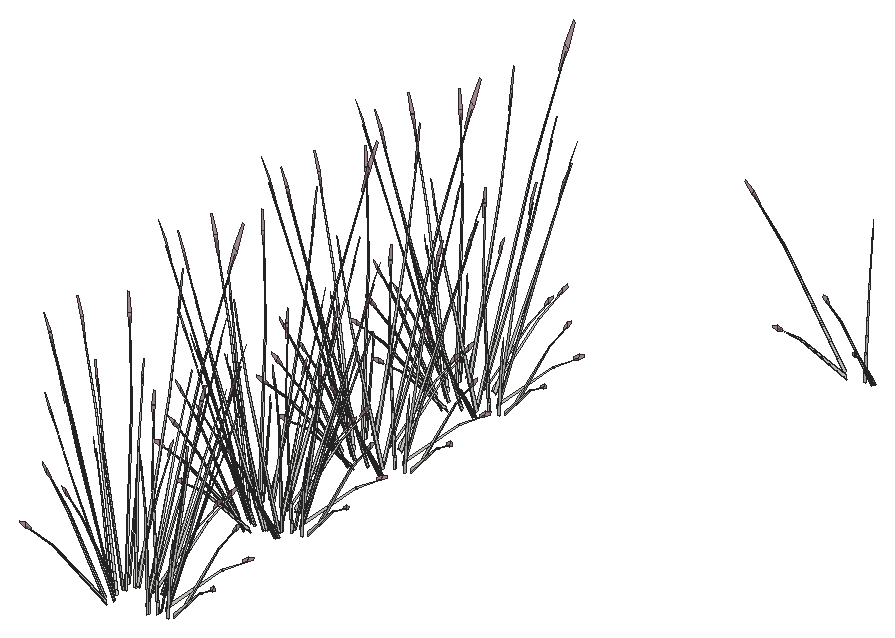
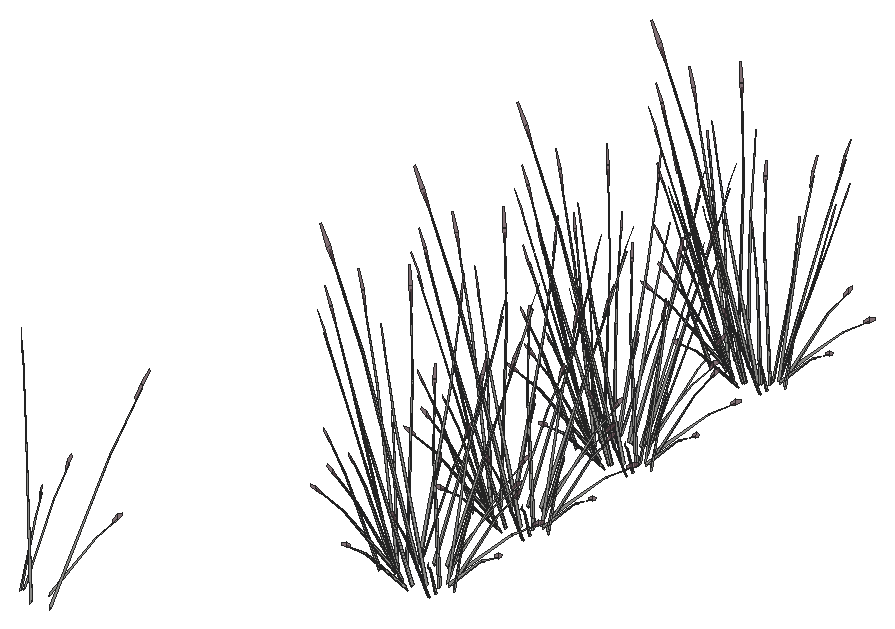
# SketchUp Ruby script. Lengths in inches.
U = 1.inch
M = Sketchup.active_model
def pt(a) = Geom::Point3d.new(a.map { |v| v * U })
def face(e, loops, mat)
  f = e.add_face(loops[0].map { |a| pt(a) })
  loops[1..].each { |l| e.add_face(l.map { |a| pt(a) }).erase! }
  f.material = f.back_material = mat if mat
  f
end
# faces: each face lists its corners as indices into pts; further lists are holes
def faces(e, pts, list, mat = nil) = list.each { |f| face(e, (f[0].is_a?(Array) ? f : [f]).map { |l| l.map { |i| pts[i] } }, mat) }
# xy, xz, yz: faces in a plane at the given z, y or x. An outline is a flat list of corners, or four numbers for a rectangle; further outlines are holes
def ring(l) = l.size == 4 ? [[l[0], l[1]], [l[2], l[1]], [l[2], l[3]], [l[0], l[3]]] : l.each_slice(2).to_a
def flat(e, list, mat, &to3) = list.each { |f| face(e, (f[0].is_a?(Array) ? f : [f]).map { |l| ring(l).map { |u, v| to3.(u, v) } }, mat) }
def xy(e, z, list, mat = nil) = flat(e, list, mat) { |x, y| [x, y, z] }
def xz(e, y, list, mat = nil) = flat(e, list, mat) { |x, z| [x, y, z] }
def yz(e, x, list, mat = nil) = flat(e, list, mat) { |y, z| [x, y, z] }
def lines(e, pts, list) = list.each { |a, b| e.add_line(pt(pts[a]), pt(pts[b])) }
# prism: a flat outline (further loops are holes) pulled along v
def prism(e, loops, v, mat = nil)
  f = face(e, loops, mat); d = Geom::Vector3d.new(v.map { |x| x * U })
  f.pushpull(f.normal.samedirection?(d) ? d.length : -d.length)
end
def box(e, o, s, mat = nil) = prism(e, [[o, [o[0] + s[0], o[1], o[2]], [o[0] + s[0], o[1] + s[1], o[2]], [o[0], o[1] + s[1], o[2]]]], [0, 0, s[2]], mat)
def at(x, y, z, deg = 0) = Geom::Transformation.translation(pt([x, y, z])) * Geom::Transformation.rotation(ORIGIN, Z_AXIS, deg.degrees)
def axes(o, x, y, z) = Geom::Transformation.new([*x, 0, *y, 0, *z, 0, *pt(o).to_a, 1])
def part(name) = M.definitions.add(name)
# library, detail: a bought-in or finely detailed component or shape, given as its bounding box
def library(name, o, s) = part(name).tap { |d| box(d.entities, o, s) }
def detail(e, o, s) = box(e.add_group.entities, o, s)
def put(e, d, t, mat = nil) = e.add_instance(d, t).tap { |i| i.material = mat if mat }
def group(e, t, mat = nil) = e.add_group.tap { |g| g.transformation = t; g.material = mat if mat }.entities
root = M.entities
M.materials.add("LightPink_Translucent").color = [144, 107, 117]
M.materials["LightPink_Translucent"].alpha = 0.75
c1 = part("blade")
p = [[2.15,0.21,22],[0,0.17,0],[0.09,0.45,0],[2.18,0.31,22],[2.29,0.31,22],[0.38,0.45,0],
  [2.48,0.24,33],[2.49,0.24,33],[2.48,0.22,33]]
faces(c1.entities,p,[[0,1,2,3],[4,5,2,3],[6,3,4,7],[8,0,3,6]])
c2 = part("seeds")
p = [[0.3,-0.1,1.38],[-0.01,-0.03,1.59],[-0.01,-0.03,0.03],[0.14,-0.07,-0.07],[0.29,-0.03,3],[0.15,0.01,3.11]]
faces(c2.entities,p,[[0,1,2,3],[1,0,4,5]],"LightPink_Translucent")
c3 = part("blade with seeds")
put(c3.entities,c1,at(0,0,0))
put(c3.entities,c2,axes([2.4,0.25,30.99],[1.5799,-0.05474,1.17369],[-0.12525,1.92788,0.29478],[-0.07173,-0.02425,1.56792]))
put(root,c3,axes([673.85,236.19,513.93],[0.53464,0.0266,0.05337],[-0.01466,0.40172,0.42015],[0.05594,-0.15388,0.64067]))
put(root,c3,axes([669.22,235.43,513.91],[-0.13998,-0.00403,1.45204],[-0.44565,0.40302,-0.22964],[-0.23779,-0.08235,0.11645]))
put(root,c3,axes([674.51,237.4375,514.18],[-0.60181,-0.31483,-0.10093],[0.34671,-0.45593,-0.56021],[0.17003,-0.15849,0.85122]))
put(root,c3,axes([675.99,237.3,513.91],[-0.08498,-0.00434,1.47228],[-0.35287,-0.46464,-0.13912],[0.14171,-0.15278,0.26054]))
put(root,c3,axes([669.37,236.34,513.93],[0.03276,-0.43418,0.05337],[0.49468,0.0119,0.42015],[-0.18949,-0.04543,0.64067]))
put(root,c3,axes([674.73,237.32,513.93],[0.44663,0.24013,0.05337],[-0.26003,0.34195,0.42015],[0.14319,-0.11055,0.64067]))
put(root,c3,axes([676.32,237.86,513.91],[0.09028,-0.08697,1.45204],[-0.11555,-0.53348,-0.22964],[0.22652,-0.10115,0.11645]))
put(root,c3,axes([668.6875,235.77,513.91],[0.04823,0.05698,1.47228],[-0.23252,0.51221,-0.13912],[-0.23548,0.00371,0.26054]))
put(root,c3,axes([669.6,236.4375,514.18],[-0.03484,0.58066,-0.10093],[-0.65957,-0.01587,-0.56021],[-0.25402,-0.04034,0.85122]))
put(root,c3,axes([674.54,238.67,514.18],[-0.32734,-0.51701,-0.10093],[0.58097,-0.25407,-0.56021],[0.24483,-0.06821,0.85122]))
put(root,c3,axes([668.6,237.52,513.93],[-0.23895,-0.38931,0.05337],[0.43573,-0.19055,0.42015],[-0.19208,0.0376,0.64067]))
put(root,c3,axes([674.8,238.65,513.93],[0.23895,0.38931,0.05337],[-0.43573,0.19055,0.42015],[0.19208,-0.0376,0.64067]))
put(root,c3,axes([675.84,240.2,513.91],[-0.05883,-0.04999,1.47228],[0.12868,-0.53581,-0.13912],[0.23172,-0.03423,0.26054]))
put(root,c3,axes([668.18,238.03,513.91],[-0.10624,0.07413,1.45204],[0.00904,0.54162,-0.22964],[-0.24352,0.07044,0.11645]))
put(root,c3,axes([668.87,237.51,514.18],[0.32734,0.51701,-0.10093],[-0.58097,0.25407,-0.56021],[-0.24483,0.06821,0.85122]))
put(root,c3,axes([673.8,239.74,514.18],[0.03484,-0.58066,-0.10093],[0.65957,0.01587,-0.56021],[0.25402,0.04034,0.85122]))
put(root,c3,axes([674.375,239.39,513.91],[0.13956,-0.00966,1.45204],[0.38281,-0.44358,-0.22964],[0.24825,0.05855,0.11645]))
put(root,c3,axes([668.67,238.86,513.93],[-0.44663,-0.24013,0.05337],[0.26003,-0.34195,0.42015],[-0.14319,0.11055,0.64067]))
put(root,c3,axes([667,238.57,513.91],[0.08303,0.01531,1.47228],[0.25685,0.50448,-0.13912],[-0.16996,0.13241,0.26054]))
put(root,c3,axes([674.04,239.84,513.93],[-0.03276,0.43418,0.05337],[-0.49468,-0.0119,0.42015],[0.18949,0.04543,0.64067]))
put(root,c3,axes([672.94,237.49,513.71],[-0.56218,-0.29666,1.14775],[0.59361,-0.46189,0.49522],[0.18138,0.27836,1.10941]))
put(root,c3,axes([668.89,238.74,514.18],[0.60181,0.31483,-0.10093],[-0.34671,0.45593,-0.56021],[-0.17003,0.15849,0.85122]))
put(root,c3,axes([672.5,240.37,514.18],[0.38768,-0.48872,-0.10093],[0.56143,0.28156,-0.56021],[0.19516,0.13808,0.85122]))
put(root,c3,axes([672,240.78,513.91],[0.00193,-0.06913,1.47228],[0.55753,-0.30498,-0.13912],[0.19366,0.10886,0.26054]))
put(root,c3,axes([669.55,239.98,513.93],[-0.53464,-0.0266,0.05337],[0.01466,-0.40172,0.42015],[-0.05594,0.15388,0.64067]))
put(root,c3,axes([672.65,240.55,513.93],[-0.29569,0.36271,0.05337],[-0.42107,-0.21117,0.42015],[0.13613,0.11629,0.64067]))
put(root,c3,axes([671,240.6,513.93],[-0.47939,0.19405,0.05337],[-0.23464,-0.35385,0.42015],[0.0463,0.15598,0.64067]))
put(root,c3,axes([668.2,240.05,513.91],[-0.01617,0.11299,1.45204],[0.45894,0.39307,-0.22964],[-0.12015,0.18588,0.11645]))
put(root,c3,axes([669.67,239.79,514.48],[0.71502,0.02829,-0.11203],[-0.01954,0.53563,-0.62183],[-0.04967,0.20629,0.94486]))
put(root,c3,axes([670.99,240.39,514.18],[0.63664,-0.26583,-0.10093],[0.31286,0.47181,-0.56021],[0.084,0.19882,0.85122]))
put(root,c3,axes([668.15,241.21,513.91],[0.07381,-0.03447,1.47228],[0.61004,0.22929,-0.13912],[-0.01434,0.19091,0.26054]))
put(root,c3,axes([670.84,241.45,513.91],[0.08247,0.09194,1.45204],[0.66552,0.03612,-0.22964],[0.06692,0.20277,0.11645]))
put(root,c3,axes([671.4,256.4,513.91],[-0.09951,-0.08005,1.45204],[-0.66407,0.05075,-0.22964],[-0.10598,-0.19148,0.11645]))
put(root,c3,axes([674.39,257.375,513.91],[-0.00628,-0.11364,1.45204],[-0.53042,-0.32843,-0.22964],[0.08201,-0.19909,0.11645]))
put(root,c3,axes([674.24,256.97,513.91],[-0.06607,0.04361,1.47228],[-0.64734,-0.14714,-0.13912],[-0.02343,-0.19032,0.26054]))
put(root,c3,axes([670.72,256.13,513.91],[-0.01214,0.06844,1.47228],[-0.59861,0.24837,-0.13912],[-0.17615,-0.12696,0.26054]))
put(root,c3,axes([672.41,257.63,514.18],[-0.63664,0.26583,-0.10093],[-0.31286,-0.47181,-0.56021],[-0.084,-0.19882,0.85122]))
put(root,c3,axes([673.74,258.23,514.18],[-0.71502,-0.02829,-0.10093],[0.01954,-0.53563,-0.56021],[0.04967,-0.20629,0.85122]))
put(root,c3,axes([672.4,257.42,513.93],[0.47939,-0.19405,0.05337],[0.23464,0.35385,0.42015],[-0.0463,-0.15598,0.64067]))
put(root,c3,axes([670.76,257.47,513.93],[0.29569,-0.36271,0.05337],[0.42107,0.21117,0.42015],[-0.13613,-0.11629,0.64067]))
put(root,c3,axes([670.89,257.43,514.51],[-0.4342,0.54737,-0.11304],[-0.6288,-0.31535,-0.62743],[-0.21858,-0.15465,0.95337]))
put(root,c3,axes([673.85,258.04,513.93],[0.53464,0.0266,0.05337],[-0.01466,0.40172,0.42015],[0.05594,-0.15388,0.64067]))
put(root,c3,axes([669.22,257.28,513.91],[-0.13998,-0.00403,1.45204],[-0.44565,0.40302,-0.22964],[-0.23779,-0.08235,0.11645]))
put(root,c3,axes([674.51,259.28,514.18],[-0.60181,-0.31483,-0.10093],[0.34671,-0.45593,-0.56021],[0.17003,-0.15849,0.85122]))
put(root,c3,axes([675.99,259.15,513.91],[-0.08498,-0.00434,1.47228],[-0.35287,-0.46464,-0.13912],[0.14171,-0.15278,0.26054]))
put(root,c3,axes([669.37,258.19,513.93],[0.03276,-0.43418,0.05337],[0.49468,0.0119,0.42015],[-0.18949,-0.04543,0.64067]))
put(root,c3,axes([674.73,259.17,513.93],[0.44663,0.24013,0.05337],[-0.26003,0.34195,0.42015],[0.14319,-0.11055,0.64067]))
put(root,c3,axes([676.32,259.7,513.91],[0.09028,-0.08697,1.45204],[-0.11555,-0.53348,-0.22964],[0.22652,-0.10115,0.11645]))
put(root,c3,axes([668.6875,257.62,513.91],[0.04823,0.05698,1.47228],[-0.23252,0.51221,-0.13912],[-0.23548,0.00371,0.26054]))
put(root,c3,axes([669.6,258.28,514.18],[-0.03484,0.58066,-0.10093],[-0.65957,-0.01587,-0.56021],[-0.25402,-0.04034,0.85122]))
put(root,c3,axes([674.54,260.51,514.18],[-0.32734,-0.51701,-0.10093],[0.58097,-0.25407,-0.56021],[0.24483,-0.06821,0.85122]))
put(root,c3,axes([674.8,260.5,513.93],[0.23895,0.38931,0.05337],[-0.43573,0.19055,0.42015],[0.19208,-0.0376,0.64067]))
put(root,c3,axes([675.84,262.05,513.91],[-0.05883,-0.04999,1.47228],[0.12868,-0.53581,-0.13912],[0.23172,-0.03423,0.26054]))
put(root,c3,axes([668.18,259.87,513.91],[-0.10624,0.07413,1.45204],[0.00904,0.54162,-0.22964],[-0.24352,0.07044,0.11645]))
put(root,c3,axes([668.87,259.36,514.18],[0.32734,0.51701,-0.10093],[-0.58097,0.25407,-0.56021],[-0.24483,0.06821,0.85122]))
put(root,c3,axes([673.8,261.58,514.18],[0.03484,-0.58066,-0.10093],[0.65957,0.01587,-0.56021],[0.25402,0.04034,0.85122]))
put(root,c3,axes([674.375,261.24,513.91],[0.13956,-0.00966,1.45204],[0.38281,-0.44358,-0.22964],[0.24825,0.05855,0.11645]))
put(root,c3,axes([668.67,260.7,513.93],[-0.44663,-0.24013,0.05337],[0.26003,-0.34195,0.42015],[-0.14319,0.11055,0.64067]))
put(root,c3,axes([667,260.42,513.91],[0.08303,0.01531,1.47228],[0.25685,0.50448,-0.13912],[-0.16996,0.13241,0.26054]))
put(root,c3,axes([674.04,261.68,513.93],[-0.03276,0.43418,0.05337],[-0.49468,-0.0119,0.42015],[0.18949,0.04543,0.64067]))
put(root,c3,axes([672.94,259.33,513.71],[-0.56218,-0.29666,1.14775],[0.59361,-0.46189,0.49522],[0.18138,0.27836,1.10941]))
put(root,c3,axes([668.89,260.58,514.18],[0.60181,0.31483,-0.10093],[-0.34671,0.45593,-0.56021],[-0.17003,0.15849,0.85122]))
put(root,c3,axes([672.5,262.22,514.18],[0.38768,-0.48872,-0.10093],[0.56143,0.28156,-0.56021],[0.19516,0.13808,0.85122]))
put(root,c3,axes([672,262.62,513.91],[0.00193,-0.06913,1.47228],[0.55753,-0.30498,-0.13912],[0.19366,0.10886,0.26054]))
put(root,c3,axes([671,262.45,513.93],[-0.47939,0.19405,0.05337],[-0.23464,-0.35385,0.42015],[0.0463,0.15598,0.64067]))
put(root,c3,axes([668.2,261.89,513.91],[-0.01617,0.11299,1.45204],[0.45894,0.39307,-0.22964],[-0.12015,0.18588,0.11645]))
put(root,c3,axes([669.67,261.64,514.48],[0.71502,0.02829,-0.11203],[-0.01954,0.53563,-0.62183],[-0.04967,0.20629,0.94486]))
put(root,c3,axes([670.99,262.24,514.18],[0.63664,-0.26583,-0.10093],[0.31286,0.47181,-0.56021],[0.084,0.19882,0.85122]))
put(root,c3,axes([668.15,263.05,513.91],[0.07381,-0.03447,1.47228],[0.61004,0.22929,-0.13912],[-0.01434,0.19091,0.26054]))
put(root,c3,axes([670.84,263.29,513.91],[0.08247,0.09194,1.45204],[0.66552,0.03612,-0.22964],[0.06692,0.20277,0.11645]))
put(root,c3,axes([671.4,273.25,513.91],[-0.09951,-0.08005,1.45204],[-0.66407,0.05075,-0.22964],[-0.10598,-0.19148,0.11645]))
put(root,c3,axes([674.39,274.24,513.91],[-0.00628,-0.11364,1.45204],[-0.53042,-0.32843,-0.22964],[0.08201,-0.19909,0.11645]))
put(root,c3,axes([674.24,273.83,513.91],[-0.06607,0.04361,1.47228],[-0.64734,-0.14714,-0.13912],[-0.02343,-0.19032,0.26054]))
put(root,c3,axes([670.72,272.99,513.91],[-0.01214,0.06844,1.47228],[-0.59861,0.24837,-0.13912],[-0.17615,-0.12696,0.26054]))
put(root,c3,axes([672.41,274.49,514.18],[-0.63664,0.26583,-0.10093],[-0.31286,-0.47181,-0.56021],[-0.084,-0.19882,0.85122]))
put(root,c3,axes([673.74,275.09,514.18],[-0.71502,-0.02829,-0.10093],[0.01954,-0.53563,-0.56021],[0.04967,-0.20629,0.85122]))
put(root,c3,axes([670.89,274.29,514.51],[-0.4342,0.54737,-0.11304],[-0.6288,-0.31535,-0.62743],[-0.21858,-0.15465,0.95337]))
put(root,c3,axes([669.22,274.14,513.91],[-0.13998,-0.00403,1.45204],[-0.44565,0.40302,-0.22964],[-0.23779,-0.08235,0.11645]))
put(root,c3,axes([674.51,276.14,514.18],[-0.60181,-0.31483,-0.10093],[0.34671,-0.45593,-0.56021],[0.17003,-0.15849,0.85122]))
put(root,c3,axes([675.99,276,513.91],[-0.08498,-0.00434,1.47228],[-0.35287,-0.46464,-0.13912],[0.14171,-0.15278,0.26054]))
put(root,c3,axes([676.32,276.56,513.91],[0.09028,-0.08697,1.45204],[-0.11555,-0.53348,-0.22964],[0.22652,-0.10115,0.11645]))
put(root,c3,axes([668.6875,274.48,513.91],[0.04823,0.05698,1.47228],[-0.23252,0.51221,-0.13912],[-0.23548,0.00371,0.26054]))
put(root,c3,axes([669.6,275.14,514.18],[-0.03484,0.58066,-0.10093],[-0.65957,-0.01587,-0.56021],[-0.25402,-0.04034,0.85122]))
put(root,c3,axes([674.54,277.37,514.18],[-0.32734,-0.51701,-0.10093],[0.58097,-0.25407,-0.56021],[0.24483,-0.06821,0.85122]))
put(root,c3,axes([675.84,278.91,513.91],[-0.05883,-0.04999,1.47228],[0.12868,-0.53581,-0.13912],[0.23172,-0.03423,0.26054]))
put(root,c3,axes([668.18,276.73,513.91],[-0.10624,0.07413,1.45204],[0.00904,0.54162,-0.22964],[-0.24352,0.07044,0.11645]))
put(root,c3,axes([668.87,276.22,514.18],[0.32734,0.51701,-0.10093],[-0.58097,0.25407,-0.56021],[-0.24483,0.06821,0.85122]))
put(root,c3,axes([673.8,278.44,514.18],[0.03484,-0.58066,-0.10093],[0.65957,0.01587,-0.56021],[0.25402,0.04034,0.85122]))
put(root,c3,axes([674.375,278.1,513.91],[0.13956,-0.00966,1.45204],[0.38281,-0.44358,-0.22964],[0.24825,0.05855,0.11645]))
put(root,c3,axes([667,277.28,513.91],[0.08303,0.01531,1.47228],[0.25685,0.50448,-0.13912],[-0.16996,0.13241,0.26054]))
put(root,c3,axes([672.94,276.19,513.71],[-0.56218,-0.29666,1.14775],[0.59361,-0.46189,0.49522],[0.18138,0.27836,1.10941]))
put(root,c3,axes([668.89,277.44,514.18],[0.60181,0.31483,-0.10093],[-0.34671,0.45593,-0.56021],[-0.17003,0.15849,0.85122]))
put(root,c3,axes([672.5,279.08,514.18],[0.38768,-0.48872,-0.10093],[0.56143,0.28156,-0.56021],[0.19516,0.13808,0.85122]))
put(root,c3,axes([672,279.48,513.91],[0.00193,-0.06913,1.47228],[0.55753,-0.30498,-0.13912],[0.19366,0.10886,0.26054]))
put(root,c3,axes([668.2,278.75,513.91],[-0.01617,0.11299,1.45204],[0.45894,0.39307,-0.22964],[-0.12015,0.18588,0.11645]))
put(root,c3,axes([669.67,278.5,514.48],[0.71502,0.02829,-0.11203],[-0.01954,0.53563,-0.62183],[-0.04967,0.20629,0.94486]))
put(root,c3,axes([670.99,279.1,514.18],[0.63664,-0.26583,-0.10093],[0.31286,0.47181,-0.56021],[0.084,0.19882,0.85122]))
put(root,c3,axes([668.15,279.91,513.91],[0.07381,-0.03447,1.47228],[0.61004,0.22929,-0.13912],[-0.01434,0.19091,0.26054]))
put(root,c3,axes([670.84,280.15,513.91],[0.08247,0.09194,1.45204],[0.66552,0.03612,-0.22964],[0.06692,0.20277,0.11645]))
put(root,c3,axes([671.4,288.59,513.91],[-0.09951,-0.08005,1.45204],[-0.66407,0.05075,-0.22964],[-0.10598,-0.19148,0.11645]))
put(root,c3,axes([674.39,289.57,513.91],[-0.00628,-0.11364,1.45204],[-0.53042,-0.32843,-0.22964],[0.08201,-0.19909,0.11645]))
put(root,c3,axes([674.24,289.16,513.91],[-0.06607,0.04361,1.47228],[-0.64734,-0.14714,-0.13912],[-0.02343,-0.19032,0.26054]))
put(root,c3,axes([670.72,288.33,513.91],[-0.01214,0.06844,1.47228],[-0.59861,0.24837,-0.13912],[-0.17615,-0.12696,0.26054]))
put(root,c3,axes([672.41,289.82,514.18],[-0.63664,0.26583,-0.10093],[-0.31286,-0.47181,-0.56021],[-0.084,-0.19882,0.85122]))
put(root,c3,axes([673.74,290.42,514.18],[-0.71502,-0.02829,-0.10093],[0.01954,-0.53563,-0.56021],[0.04967,-0.20629,0.85122]))
put(root,c3,axes([670.89,289.63,514.51],[-0.4342,0.54737,-0.11304],[-0.6288,-0.31535,-0.62743],[-0.21858,-0.15465,0.95337]))
put(root,c3,axes([669.22,289.47,513.91],[-0.13998,-0.00403,1.45204],[-0.44565,0.40302,-0.22964],[-0.23779,-0.08235,0.11645]))
put(root,c3,axes([674.51,291.48,514.18],[-0.60181,-0.31483,-0.10093],[0.34671,-0.45593,-0.56021],[0.17003,-0.15849,0.85122]))
put(root,c3,axes([675.99,291.34,513.91],[-0.08498,-0.00434,1.47228],[-0.35287,-0.46464,-0.13912],[0.14171,-0.15278,0.26054]))
put(root,c3,axes([676.32,291.89,513.91],[0.09028,-0.08697,1.45204],[-0.11555,-0.53348,-0.22964],[0.22652,-0.10115,0.11645]))
put(root,c3,axes([668.6875,289.8125,513.91],[0.04823,0.05698,1.47228],[-0.23252,0.51221,-0.13912],[-0.23548,0.00371,0.26054]))
put(root,c3,axes([669.6,290.48,514.18],[-0.03484,0.58066,-0.10093],[-0.65957,-0.01587,-0.56021],[-0.25402,-0.04034,0.85122]))
put(root,c3,axes([674.54,292.7,514.18],[-0.32734,-0.51701,-0.10093],[0.58097,-0.25407,-0.56021],[0.24483,-0.06821,0.85122]))
put(root,c3,axes([675.84,294.24,513.91],[-0.05883,-0.04999,1.47228],[0.12868,-0.53581,-0.13912],[0.23172,-0.03423,0.26054]))
put(root,c3,axes([668.18,292.07,513.91],[-0.10624,0.07413,1.45204],[0.00904,0.54162,-0.22964],[-0.24352,0.07044,0.11645]))
put(root,c3,axes([668.87,291.55,514.18],[0.32734,0.51701,-0.10093],[-0.58097,0.25407,-0.56021],[-0.24483,0.06821,0.85122]))
put(root,c3,axes([673.8,293.78,514.18],[0.03484,-0.58066,-0.10093],[0.65957,0.01587,-0.56021],[0.25402,0.04034,0.85122]))
put(root,c3,axes([674.375,293.43,513.91],[0.13956,-0.00966,1.45204],[0.38281,-0.44358,-0.22964],[0.24825,0.05855,0.11645]))
put(root,c3,axes([667,292.61,513.91],[0.08303,0.01531,1.47228],[0.25685,0.50448,-0.13912],[-0.16996,0.13241,0.26054]))
put(root,c3,axes([672.94,291.53,513.71],[-0.56218,-0.29666,1.14775],[0.59361,-0.46189,0.49522],[0.18138,0.27836,1.10941]))
put(root,c3,axes([668.89,292.78,514.18],[0.60181,0.31483,-0.10093],[-0.34671,0.45593,-0.56021],[-0.17003,0.15849,0.85122]))
put(root,c3,axes([672.5,294.41,514.18],[0.38768,-0.48872,-0.10093],[0.56143,0.28156,-0.56021],[0.19516,0.13808,0.85122]))
put(root,c3,axes([672,294.82,513.91],[0.00193,-0.06913,1.47228],[0.55753,-0.30498,-0.13912],[0.19366,0.10886,0.26054]))
put(root,c3,axes([668.2,294.09,513.91],[-0.01617,0.11299,1.45204],[0.45894,0.39307,-0.22964],[-0.12015,0.18588,0.11645]))
put(root,c3,axes([669.67,293.83,514.48],[0.71502,0.02829,-0.11203],[-0.01954,0.53563,-0.62183],[-0.04967,0.20629,0.94486]))
put(root,c3,axes([670.99,294.43,514.18],[0.63664,-0.26583,-0.10093],[0.31286,0.47181,-0.56021],[0.084,0.19882,0.85122]))
put(root,c3,axes([668.15,295.25,513.91],[0.07381,-0.03447,1.47228],[0.61004,0.22929,-0.13912],[-0.01434,0.19091,0.26054]))
put(root,c3,axes([670.84,295.49,513.91],[0.08247,0.09194,1.45204],[0.66552,0.03612,-0.22964],[0.06692,0.20277,0.11645]))
put(root,c3,axes([697.87,320.5,513.22],[0.14872,0.18332,1.42242],[-0.6872,0.15433,0.11501],[-0.15531,-0.28779,0.60807]))
put(root,c3,axes([699.01,319.28,513.91],[-0.09951,-0.08005,1.45204],[-0.66407,0.05075,-0.22964],[-0.10598,-0.19148,0.11645]))
put(root,c3,axes([701.99,320.26,513.91],[-0.00628,-0.11364,1.45204],[-0.53042,-0.32843,-0.22964],[0.08201,-0.19909,0.11645]))
put(root,c3,axes([700.19,320.82,513.22],[-0.12114,0.19625,1.42242],[-0.50818,-0.40613,0.11501],[0.22925,-0.25313,0.60807]))
put(root,c3,axes([701.85,319.85,513.91],[-0.06607,0.04361,1.47228],[-0.64734,-0.14714,-0.13912],[-0.02343,-0.19032,0.26054]))
